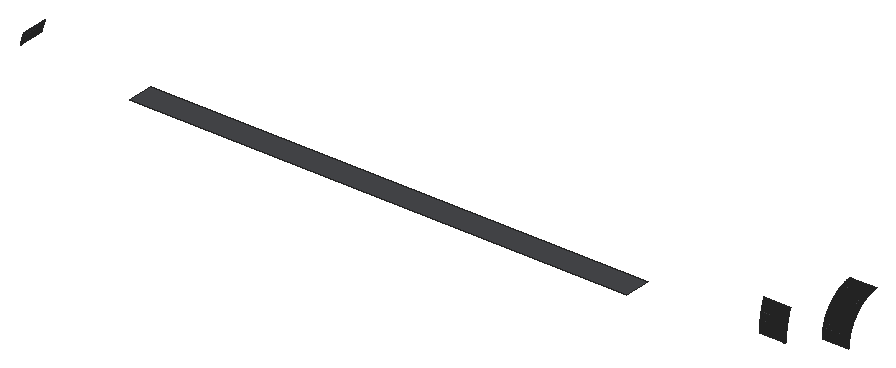
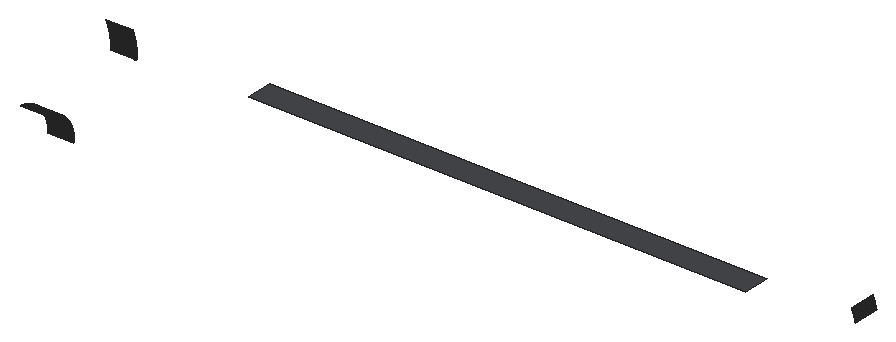
# SketchUp Ruby script. Lengths in inches.
U = 1.inch
M = Sketchup.active_model
def pt(a) = Geom::Point3d.new(a.map { |v| v * U })
def face(e, loops, mat)
  f = e.add_face(loops[0].map { |a| pt(a) })
  loops[1..].each { |l| e.add_face(l.map { |a| pt(a) }).erase! }
  f.material = f.back_material = mat if mat
  f
end
# faces: each face lists its corners as indices into pts; further lists are holes
def faces(e, pts, list, mat = nil) = list.each { |f| face(e, (f[0].is_a?(Array) ? f : [f]).map { |l| l.map { |i| pts[i] } }, mat) }
# xy, xz, yz: faces in a plane at the given z, y or x. An outline is a flat list of corners, or four numbers for a rectangle; further outlines are holes
def ring(l) = l.size == 4 ? [[l[0], l[1]], [l[2], l[1]], [l[2], l[3]], [l[0], l[3]]] : l.each_slice(2).to_a
def flat(e, list, mat, &to3) = list.each { |f| face(e, (f[0].is_a?(Array) ? f : [f]).map { |l| ring(l).map { |u, v| to3.(u, v) } }, mat) }
def xy(e, z, list, mat = nil) = flat(e, list, mat) { |x, y| [x, y, z] }
def xz(e, y, list, mat = nil) = flat(e, list, mat) { |x, z| [x, y, z] }
def yz(e, x, list, mat = nil) = flat(e, list, mat) { |y, z| [x, y, z] }
def lines(e, pts, list) = list.each { |a, b| e.add_line(pt(pts[a]), pt(pts[b])) }
# prism: a flat outline (further loops are holes) pulled along v
def prism(e, loops, v, mat = nil)
  f = face(e, loops, mat); d = Geom::Vector3d.new(v.map { |x| x * U })
  f.pushpull(f.normal.samedirection?(d) ? d.length : -d.length)
end
def box(e, o, s, mat = nil) = prism(e, [[o, [o[0] + s[0], o[1], o[2]], [o[0] + s[0], o[1] + s[1], o[2]], [o[0], o[1] + s[1], o[2]]]], [0, 0, s[2]], mat)
def at(x, y, z, deg = 0) = Geom::Transformation.translation(pt([x, y, z])) * Geom::Transformation.rotation(ORIGIN, Z_AXIS, deg.degrees)
def axes(o, x, y, z) = Geom::Transformation.new([*x, 0, *y, 0, *z, 0, *pt(o).to_a, 1])
def part(name) = M.definitions.add(name)
# library, detail: a bought-in or finely detailed component or shape, given as its bounding box
def library(name, o, s) = part(name).tap { |d| box(d.entities, o, s) }
def detail(e, o, s) = box(e.add_group.entities, o, s)
def put(e, d, t, mat = nil) = e.add_instance(d, t).tap { |i| i.material = mat if mat }
def group(e, t, mat = nil) = e.add_group.tap { |g| g.transformation = t; g.material = mat if mat }.entities
root = M.entities
M.materials.add("1432 AP 8245 TAR ROAD").color = [71, 72, 75]
xy(root,563.79,[[294,95.37,522,107.37]],"1432 AP 8245 TAR ROAD")
xz(root,107.37,[[573,560.79,585,561.07]],"1432 AP 8245 TAR ROAD")
xz(root,143.37,[[573,542.79,585,543.03]],"1432 AP 8245 TAR ROAD")
p = [[573,143.37,543.03],[573,143.375,543.26],[585,143.375,543.26],[585,143.37,543.03],[573,143.38,543.5],[585,143.38,543.5],
  [573,143.39,543.73],[585,143.39,543.73],[573,143.41,543.97],[585,143.41,543.97],[573,143.43,544.2],[585,143.43,544.2],
  [573,143.45,544.4375],[585,143.45,544.4375],[573,143.47,544.67],[585,143.47,544.67],[573,143.49,544.91],[585,143.49,544.91],
  [573,143.52,545.14],[585,143.52,545.14],[573,143.56,545.375],[585,143.56,545.375],[573,143.59,545.61],[585,143.59,545.61],
  [573,143.63,545.84],[585,143.63,545.84],[573,143.67,546.07],[585,143.67,546.07],[573,143.72,546.3],[585,143.72,546.3],
  [573,143.76,546.53],[585,143.76,546.53],[573,143.8125,546.76],[585,143.8125,546.76],[573,143.87,546.99],[585,143.87,546.99],
  [573,143.92,547.22],[585,143.92,547.22],[573,143.98,547.45],[585,143.98,547.45],[573,144.05,547.68],[585,144.05,547.68],
  [573,144.11,547.9],[585,144.11,547.9],[573,144.18,548.13],[585,144.18,548.13],[573,144.25,548.35],[585,144.25,548.35],
  [573,144.33,548.58],[585,144.33,548.58],[573,144.4,548.8],[585,144.4,548.8],[573,144.48,549.02],[585,144.48,549.02],
  [573,144.57,549.24],[585,144.57,549.24],[573,144.65,549.46],[585,144.65,549.46],[573,144.74,549.68],[585,144.74,549.68],
  [573,144.83,549.9],[585,144.83,549.9],[573,144.93,550.11],[585,144.93,550.11],[573,145.02,550.33],[585,145.02,550.33],
  [573,145.125,550.54],[585,145.125,550.54],[573,145.23,550.75],[585,145.23,550.75],[573,145.33,550.96],[585,145.33,550.96],
  [573,145.44,551.17],[585,145.44,551.17],[573,145.55,551.38],[585,145.55,551.38],[573,145.67,551.59],[585,145.67,551.59],
  [573,145.78,551.79],[585,145.78,551.79],[573,145.9,552],[585,145.9,552],[573,146.02,552.2],[585,146.02,552.2],
  [573,146.15,552.4],[585,146.15,552.4],[573,146.27,552.6],[585,146.27,552.6],[573,146.4,552.79],[585,146.4,552.79],
  [573,146.54,552.99],[585,146.54,552.99],[573,146.67,553.18],[585,146.67,553.18],[573,146.81,553.37],[585,146.81,553.37],
  [573,146.95,553.5625],[585,146.95,553.5625],[573,147.09,553.75],[585,147.09,553.75],[573,147.23,553.9375],[585,147.23,553.9375],
  [573,147.38,554.12],[585,147.38,554.12],[573,147.53,554.3],[585,147.53,554.3],[573,147.68,554.48],[585,147.68,554.48],
  [573,147.84,554.66],[585,147.84,554.66],[573,147.99,554.84],[585,147.99,554.84],[573,148.15,555.01],[585,148.15,555.01],
  [573,148.3125,555.18],[585,148.3125,555.18],[573,148.48,555.35],[585,148.48,555.35],[573,148.64,555.52],[585,148.64,555.52],
  [573,148.81,555.69],[585,148.81,555.69],[573,148.98,555.85],[585,148.98,555.85],[573,149.15,556.01],[585,149.15,556.01],
  [573,149.33,556.17],[585,149.33,556.17],[573,149.5,556.33],[585,149.5,556.33],[573,149.68,556.48],[585,149.68,556.48],
  [573,149.86,556.63],[585,149.86,556.63],[573,150.04,556.78],[585,150.04,556.78],[573,150.23,556.93],[585,150.23,556.93],
  [573,150.41,557.07],[585,150.41,557.07],[573,150.6,557.21],[585,150.6,557.21],[573,150.79,557.35],[585,150.79,557.35],
  [573,150.98,557.49],[585,150.98,557.49],[573,151.17,557.625],[585,151.17,557.625],[573,151.37,557.76],[585,151.37,557.76],
  [573,151.57,557.89],[585,151.57,557.89],[573,151.76,558.02],[585,151.76,558.02],[573,151.96,558.14],[585,151.96,558.14],
  [573,152.17,558.26],[585,152.17,558.26],[573,152.37,558.38],[585,152.37,558.38],[573,152.57,558.5],[585,152.57,558.5],
  [573,152.78,558.61],[585,152.78,558.61],[573,152.99,558.72],[585,152.99,558.72],[573,153.2,558.83],[585,153.2,558.83],
  [573,153.41,558.9375],[585,153.41,558.9375],[573,153.62,559.04],[585,153.62,559.04],[573,153.83,559.14],[585,153.83,559.14],
  [573,154.05,559.24],[585,154.05,559.24],[573,154.26,559.33],[585,154.26,559.33],[573,154.48,559.42],[585,154.48,559.42],
  [573,154.7,559.51],[585,154.7,559.51],[573,154.92,559.6],[585,154.92,559.6],[573,155.14,559.68],[585,155.14,559.68],
  [573,155.36,559.76],[585,155.36,559.76],[573,155.58,559.84],[585,155.58,559.84],[573,155.81,559.91],[585,155.81,559.91],
  [573,156.03,559.98],[585,156.03,559.98],[573,156.26,560.05],[585,156.26,560.05],[573,156.48,560.12],[585,156.48,560.12],
  [573,156.71,560.18],[585,156.71,560.18],[573,156.9375,560.24],[585,156.9375,560.24],[573,157.17,560.29],[585,157.17,560.29],
  [573,157.4,560.35],[585,157.4,560.35],[573,157.63,560.4],[585,157.63,560.4],[573,157.86,560.45],[585,157.86,560.45],
  [573,158.09,560.49],[585,158.09,560.49],[573,158.32,560.53],[585,158.32,560.53],[573,158.55,560.57],[585,158.55,560.57],
  [573,158.79,560.61],[585,158.79,560.61],[573,159.02,560.64],[585,159.02,560.64],[573,159.25,560.67],[585,159.25,560.67],
  [573,107.375,561.36],[573,107.37,561.07],[585,107.37,561.07],[585,107.375,561.36],[573,107.38,561.64],[585,107.38,561.64],
  [573,107.39,561.92],[585,107.39,561.92],[573,107.4,562.21],[585,107.4,562.21],[573,107.41,562.49],[585,107.41,562.49],
  [573,107.42,562.77],[585,107.42,562.77],[573,107.44,563.05],[585,107.44,563.05],[573,107.46,563.33],[585,107.46,563.33],
  [573,107.48,563.62],[585,107.48,563.62],[573,107.5,563.9],[585,107.5,563.9],[573,107.53,564.18],[585,107.53,564.18],
  [573,107.56,564.46],[585,107.56,564.46],[573,107.59,564.74],[585,107.59,564.74],[573,107.62,565.02],[585,107.62,565.02],
  [573,107.65,565.3],[585,107.65,565.3],[573,107.69,565.58],[585,107.69,565.58],[573,107.73,565.86],[585,107.73,565.86],
  [573,107.77,566.14],[585,107.77,566.14],[573,107.8125,566.42],[585,107.8125,566.42],[573,107.86,566.7],[585,107.86,566.7],
  [573,107.91,566.98],[585,107.91,566.98],[573,107.96,567.26],[585,107.96,567.26],[573,108.01,567.54],[585,108.01,567.54],
  [573,108.0625,567.82],[585,108.0625,567.82],[573,108.12,568.09],[585,108.12,568.09],[573,108.18,568.37],[585,108.18,568.37],
  [573,108.24,568.65],[585,108.24,568.65],[243.93,107.37,568.92],[243.87,107.37,568.65],[243.87,95.37,568.65],[243.93,95.37,568.92],
  [573,108.3,568.92],[585,108.3,568.92],[243.99,107.37,569.2],[243.99,95.37,569.2],[573,108.36,569.2],[585,108.36,569.2],
  [244.0625,107.37,569.47],[244.0625,95.37,569.47],[573,108.43,569.47],[585,108.43,569.47],[244.13,107.37,569.74],[244.13,95.37,569.74],
  [573,108.5,569.74],[585,108.5,569.74],[244.2,107.37,570.02],[244.2,95.37,570.02],[573,108.57,570.02],[585,108.57,570.02],
  [244.28,107.37,570.29],[244.28,95.37,570.29],[573,108.65,570.29],[585,108.65,570.29],[244.35,107.37,570.5625],[244.35,95.37,570.5625],
  [573,108.72,570.5625],[585,108.72,570.5625],[244.43,107.37,570.84],[244.43,95.37,570.84],[573,108.8,570.84],[585,108.8,570.84],
  [244.51,107.37,571.11],[244.51,95.37,571.11],[573,108.88,571.11],[585,108.88,571.11],[244.59,107.37,571.38],[244.59,95.37,571.38],
  [573,108.96,571.38],[585,108.96,571.38],[244.68,107.37,571.65],[244.68,95.37,571.65],[573,109.05,571.65],[585,109.05,571.65],
  [244.76,107.37,571.92],[244.76,95.37,571.92],[573,109.13,571.92],[585,109.13,571.92],[244.85,107.37,572.19],[244.85,95.37,572.19],
  [573,109.22,572.19],[585,109.22,572.19],[244.94,107.37,572.45],[244.94,95.37,572.45],[573,109.3125,572.45],[585,109.3125,572.45],
  [245.03,107.37,572.72],[245.03,95.37,572.72],[573,109.4,572.72],[585,109.4,572.72],[245.13,107.37,572.99],[245.13,95.37,572.99],
  [573,109.5,572.99],[585,109.5,572.99],[245.23,107.37,573.25],[245.23,95.37,573.25],[573,109.6,573.25],[585,109.6,573.25],
  [245.32,107.37,573.52],[245.32,95.37,573.52],[573,109.69,573.52],[585,109.69,573.52],[245.42,107.37,573.78],[245.42,95.37,573.78],
  [573,109.79,573.78],[585,109.79,573.78],[245.53,107.37,574.04],[245.53,95.37,574.04],[573,109.9,574.04],[585,109.9,574.04],
  [245.63,107.37,574.31],[245.63,95.37,574.31],[573,110,574.31],[585,110,574.31]]
faces(root,p,[[0,1,2,3],[1,4,5,2],[4,6,7,5],[6,8,9,7],[8,10,11,9],[10,12,13,11],[12,14,15,13],[14,16,17,15],
  [16,18,19,17],[18,20,21,19],[20,22,23,21],[22,24,25,23],[24,26,27,25],[26,28,29,27],[28,30,31,29],[30,32,33,31],
  [32,34,35,33],[34,36,37,35],[36,38,39,37],[38,40,41,39],[40,42,43,41],[42,44,45,43],[44,46,47,45],[46,48,49,47],
  [48,50,51,49],[50,52,53,51],[52,54,55,53],[54,56,57,55],[56,58,59,57],[58,60,61,59],[60,62,63,61],[62,64,65,63],
  [64,66,67,65],[66,68,69,67],[68,70,71,69],[70,72,73,71],[72,74,75,73],[74,76,77,75],[76,78,79,77],[78,80,81,79],
  [80,82,83,81],[82,84,85,83],[84,86,87,85],[86,88,89,87],[88,90,91,89],[90,92,93,91],[92,94,95,93],[94,96,97,95],
  [96,98,99,97],[98,100,101,99],[100,102,103,101],[102,104,105,103],[104,106,107,105],[106,108,109,107],[108,110,111,109],[110,112,113,111],
  [112,114,115,113],[114,116,117,115],[116,118,119,117],[118,120,121,119],[120,122,123,121],[122,124,125,123],[124,126,127,125],[126,128,129,127],
  [128,130,131,129],[130,132,133,131],[132,134,135,133],[134,136,137,135],[136,138,139,137],[138,140,141,139],[140,142,143,141],[142,144,145,143],
  [144,146,147,145],[146,148,149,147],[148,150,151,149],[150,152,153,151],[152,154,155,153],[154,156,157,155],[156,158,159,157],[158,160,161,159],
  [160,162,163,161],[162,164,165,163],[164,166,167,165],[166,168,169,167],[168,170,171,169],[170,172,173,171],[172,174,175,173],[174,176,177,175],
  [176,178,179,177],[178,180,181,179],[180,182,183,181],[182,184,185,183],[184,186,187,185],[186,188,189,187],[188,190,191,189],[190,192,193,191],
  [192,194,195,193],[194,196,197,195],[196,198,199,197],[198,200,201,199],[200,202,203,201],[202,204,205,203],[204,206,207,205],[206,208,209,207],
  [208,210,211,209],[210,212,213,211],[212,214,215,213],[214,216,217,215],[216,218,219,217],[218,220,221,219],[222,223,224,225],[226,222,225,227],
  [228,226,227,229],[230,228,229,231],[232,230,231,233],[234,232,233,235],[236,234,235,237],[238,236,237,239],[240,238,239,241],[242,240,241,243],
  [244,242,243,245],[246,244,245,247],[248,246,247,249],[250,248,249,251],[252,250,251,253],[254,252,253,255],[256,254,255,257],[258,256,257,259],
  [260,258,259,261],[262,260,261,263],[264,262,263,265],[266,264,265,267],[268,266,267,269],[270,268,269,271],[272,270,271,273],[274,272,273,275],
  [276,274,275,277],[278,279,280,281],[282,276,277,283],[284,278,281,285],[286,282,283,287],[288,284,285,289],[290,286,287,291],[292,288,289,293],
  [294,290,291,295],[296,292,293,297],[298,294,295,299],[300,296,297,301],[302,298,299,303],[304,300,301,305],[306,302,303,307],[308,304,305,309],
  [310,306,307,311],[312,308,309,313],[314,310,311,315],[316,312,313,317],[318,314,315,319],[320,316,317,321],[322,318,319,323],[324,320,321,325],
  [326,322,323,327],[328,324,325,329],[330,326,327,331],[332,328,329,333],[334,330,331,335],[336,332,333,337],[338,334,335,339],[340,336,337,341],
  [342,338,339,343],[344,340,341,345],[346,342,343,347],[348,344,345,349],[350,346,347,351],[352,348,349,353],[354,350,351,355],[356,352,353,357],
  [358,354,355,359],[360,356,357,361],[362,358,359,363]],"1432 AP 8245 TAR ROAD")
